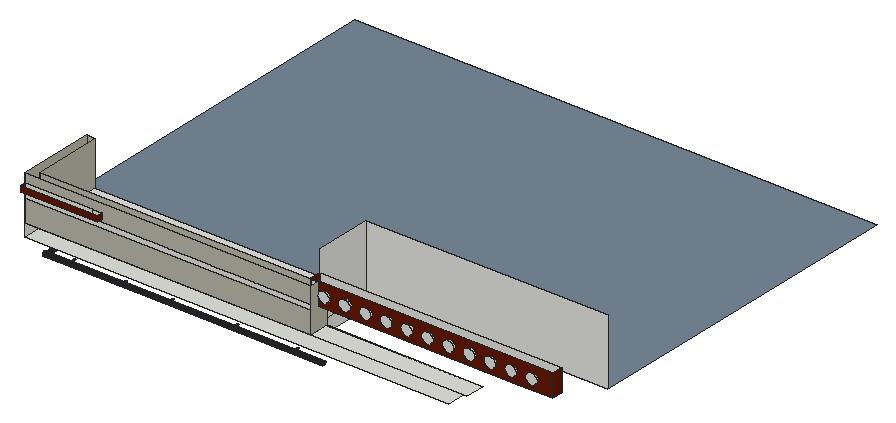
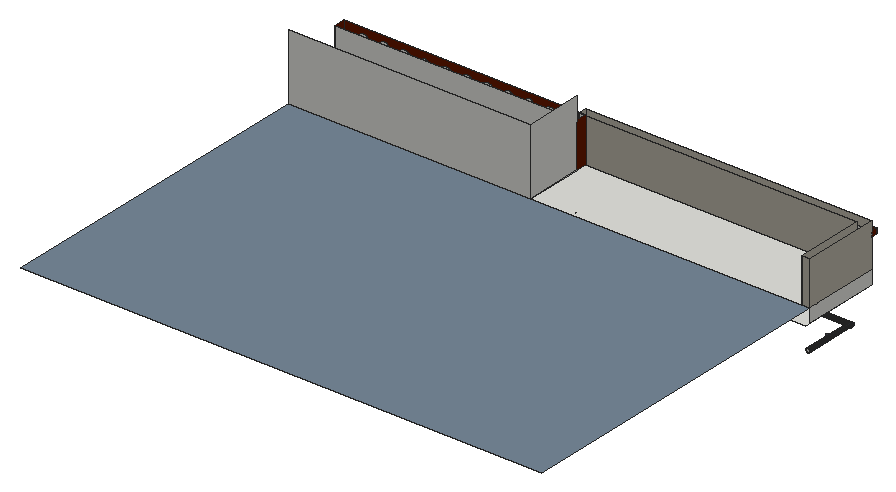
# SketchUp Ruby script. Lengths in inches.
U = 1.inch
M = Sketchup.active_model
def pt(a) = Geom::Point3d.new(a.map { |v| v * U })
def face(e, loops, mat)
  f = e.add_face(loops[0].map { |a| pt(a) })
  loops[1..].each { |l| e.add_face(l.map { |a| pt(a) }).erase! }
  f.material = f.back_material = mat if mat
  f
end
# faces: each face lists its corners as indices into pts; further lists are holes
def faces(e, pts, list, mat = nil) = list.each { |f| face(e, (f[0].is_a?(Array) ? f : [f]).map { |l| l.map { |i| pts[i] } }, mat) }
# xy, xz, yz: faces in a plane at the given z, y or x. An outline is a flat list of corners, or four numbers for a rectangle; further outlines are holes
def ring(l) = l.size == 4 ? [[l[0], l[1]], [l[2], l[1]], [l[2], l[3]], [l[0], l[3]]] : l.each_slice(2).to_a
def flat(e, list, mat, &to3) = list.each { |f| face(e, (f[0].is_a?(Array) ? f : [f]).map { |l| ring(l).map { |u, v| to3.(u, v) } }, mat) }
def xy(e, z, list, mat = nil) = flat(e, list, mat) { |x, y| [x, y, z] }
def xz(e, y, list, mat = nil) = flat(e, list, mat) { |x, z| [x, y, z] }
def yz(e, x, list, mat = nil) = flat(e, list, mat) { |y, z| [x, y, z] }
def lines(e, pts, list) = list.each { |a, b| e.add_line(pt(pts[a]), pt(pts[b])) }
# prism: a flat outline (further loops are holes) pulled along v
def prism(e, loops, v, mat = nil)
  f = face(e, loops, mat); d = Geom::Vector3d.new(v.map { |x| x * U })
  f.pushpull(f.normal.samedirection?(d) ? d.length : -d.length)
end
def box(e, o, s, mat = nil) = prism(e, [[o, [o[0] + s[0], o[1], o[2]], [o[0] + s[0], o[1] + s[1], o[2]], [o[0], o[1] + s[1], o[2]]]], [0, 0, s[2]], mat)
def at(x, y, z, deg = 0) = Geom::Transformation.translation(pt([x, y, z])) * Geom::Transformation.rotation(ORIGIN, Z_AXIS, deg.degrees)
def axes(o, x, y, z) = Geom::Transformation.new([*x, 0, *y, 0, *z, 0, *pt(o).to_a, 1])
def part(name) = M.definitions.add(name)
# library, detail: a bought-in or finely detailed component or shape, given as its bounding box
def library(name, o, s) = part(name).tap { |d| box(d.entities, o, s) }
def detail(e, o, s) = box(e.add_group.entities, o, s)
def put(e, d, t, mat = nil) = e.add_instance(d, t).tap { |i| i.material = mat if mat }
def group(e, t, mat = nil) = e.add_group.tap { |g| g.transformation = t; g.material = mat if mat }.entities
root = M.entities
M.materials.add("[0110_LightSlateGray]").color = [119, 136, 153]
M.materials.add("[0137_Black]").color = [0, 0, 0]
M.materials.add("[Color B08]").color = [102, 25, 0]
M.materials.add("[Formica Graystone]1").color = [186, 182, 168]
M.materials.add("[Formica Laminate Dark]").color = [50, 53, 60]
M.materials.add("[Wood Veneer 01]").color = [120, 70, 37]
xy(root,441.65,[[6.47,233.53,6.73,233.57,6.97,233.67,7.17,233.83,7.33,234.03,7.43,234.28,7.47,234.53,7.43,234.79,7.33,235.03,7.17,235.24,6.97,235.4,6.73,235.5,6.47,235.53,6.21,235.5,5.97,235.4,5.76,235.24,5.6,235.03,5.5,234.79,5.47,234.53,5.5,234.28,5.6,234.03,5.76,233.83,5.97,233.67,6.21,233.57]],"[Formica Laminate Dark]")
xy(root,442.09,[[91.52,203.04,91.78,203.07,92.02,203.17,92.22,203.33,92.38,203.54,92.48,203.78,92.52,204.04,92.48,204.3,92.38,204.54,92.22,204.75,92.02,204.91,91.78,205.01,91.52,205.04,91.26,205.01,91.02,204.91,90.81,204.75,90.65,204.54,90.55,204.3,90.52,204.04,90.55,203.78,90.65,203.54,90.81,203.33,91.02,203.17,91.26,203.07],[142.52,203.04,142.78,203.07,143.02,203.17,143.22,203.33,143.38,203.54,143.48,203.78,143.52,204.04,143.48,204.3,143.38,204.54,143.22,204.75,143.02,204.91,142.78,205.01,142.52,205.04,142.26,205.01,142.02,204.91,141.81,204.75,141.65,204.54,141.55,204.3,141.52,204.04,141.55,203.78,141.65,203.54,141.81,203.33,142.02,203.17,142.26,203.07],[212.89,203.04,213.15,203.07,213.39,203.17,213.6,203.33,213.76,203.54,213.86,203.78,213.89,204.04,213.86,204.3,213.76,204.54,213.6,204.75,213.39,204.91,213.15,205.01,212.89,205.04,212.63,205.01,212.39,204.91,212.18,204.75,212.03,204.54,211.93,204.3,211.89,204.04,211.93,203.78,212.03,203.54,212.18,203.33,212.39,203.17,212.63,203.07],[278.52,203.04,278.78,203.07,279.02,203.17,279.22,203.33,279.38,203.54,279.48,203.78,279.52,204.04,279.48,204.3,279.38,204.54,279.22,204.75,279.02,204.91,278.78,205.01,278.52,205.04,278.26,205.01,278.02,204.91,277.81,204.75,277.65,204.54,277.55,204.3,277.52,204.04,277.55,203.78,277.65,203.54,277.81,203.33,278.02,203.17,278.26,203.07],[34.52,204.5,34.78,204.53,35.02,204.63,35.23,204.79,35.39,205,35.49,205.24,35.52,205.5,35.49,205.76,35.39,206,35.23,206.21,35.02,206.37,34.78,206.47,34.52,206.5,34.26,206.47,34.02,206.37,33.82,206.21,33.66,206,33.56,205.76,33.52,205.5,33.56,205.24,33.66,205,33.82,204.79,34.02,204.63,34.26,204.53]],"[Formica Laminate Dark]")
xy(root,443.01,[[181.09,258.0625,209.84,261.0625],[212.72,258.0625,232.97,261.0625]])
xy(root,446.01,[[178.09,258.0625,235.97,261.0625]],"[0137_Black]")
xy(root,454.9,[[101.3,255.0625,149.3,261.0625]],"[Wood Veneer 01]")
xy(root,460.9,[[95.3,255.0625,155.3,261.0625]],"[Wood Veneer 01]")
xy(root,465.86,[[3.53,177.0625,3.53,267.0625,307.22,267.0625,307.22,198.0625,464.34,198.0625,464.34,177.0625]])
xy(root,480,[[3.53,177.0625,3.53,261.0625,12.53,261.0625,12.53,186.0625,314.59,186.0625,314.59,177.0625],[314.59,177.0625,483.9,198.0625],[12.53,186.0625,307.22,261.0625]])
xy(root,480,[[3.53,261.0625,569.78,625.1875]],"[0110_LightSlateGray]")
xy(root,504.07,[[534.65,186.0625,569.78,198.0625]])
xy(root,504.07,[[314.59,186.0625,534.65,198.0625]],"[Color B08]")
xy(root,512.39,[[3.53,171.0625,87.4,177.0625]],"[Color B08]")
xz(root,171.0625,[[3.53,512.39,87.4,518.76]],"[Color B08]")
xz(root,177.0625,[[3.53,504,314.59,509.53],[3.53,512.39,76.9,518.76],[76.9,512.39,87.4,518.76]])
xz(root,177.0625,[[3.53,480,314.59,504],[3.53,509.53,314.59,509.53,314.59,528,3.53,528,3.53,518.76,87.4,518.76,87.4,512.39,3.53,512.39]],"[Formica Graystone]1")
xz(root,183.0625,[[323.11,510.74,324.6,510.93,325.99,511.51,327.18,512.42,328.09,513.61,328.66,515,328.86,516.49,328.66,517.97,328.09,519.36,327.18,520.55,325.99,521.46,324.6,522.04,323.11,522.24,321.62,522.04,320.24,521.46,319.04,520.55,318.13,519.36,317.56,517.97,317.36,516.49,317.56,515,318.13,513.61,319.04,512.42,320.24,511.51,321.62,510.93],[345.67,510.74,347.16,510.93,348.55,511.51,349.74,512.42,350.65,513.61,351.23,515,351.42,516.49,351.23,517.97,350.65,519.36,349.74,520.55,348.55,521.46,347.16,522.04,345.67,522.24,344.19,522.04,342.8,521.46,341.61,520.55,340.69,519.36,340.12,517.97,339.92,516.49,340.12,515,340.69,513.61,341.61,512.42,342.8,511.51,344.19,510.93],[368.24,510.74,369.72,510.93,371.11,511.51,372.3,512.42,373.22,513.61,373.79,515,373.99,516.49,373.79,517.97,373.22,519.36,372.3,520.55,371.11,521.46,369.72,522.04,368.24,522.24,366.75,522.04,365.36,521.46,364.17,520.55,363.26,519.36,362.68,517.97,362.49,516.49,362.68,515,363.26,513.61,364.17,512.42,365.36,511.51,366.75,510.93],[390.8,510.74,392.29,510.93,393.67,511.51,394.86,512.42,395.78,513.61,396.35,515,396.55,516.49,396.35,517.97,395.78,519.36,394.86,520.55,393.67,521.46,392.29,522.04,390.8,522.24,389.31,522.04,387.92,521.46,386.73,520.55,385.82,519.36,385.24,517.97,385.05,516.49,385.24,515,385.82,513.61,386.73,512.42,387.92,511.51,389.31,510.93],[413.36,510.74,414.85,510.93,416.24,511.51,417.43,512.42,418.34,513.61,418.91,515,419.11,516.49,418.91,517.97,418.34,519.36,417.43,520.55,416.24,521.46,414.85,522.04,413.36,522.24,411.87,522.04,410.49,521.46,409.29,520.55,408.38,519.36,407.81,517.97,407.61,516.49,407.81,515,408.38,513.61,409.29,512.42,410.49,511.51,411.87,510.93],
  [435.92,510.74,437.41,510.93,438.8,511.51,439.99,512.42,440.9,513.61,441.48,515,441.67,516.49,441.48,517.97,440.9,519.36,439.99,520.55,438.8,521.46,437.41,522.04,435.92,522.24,434.44,522.04,433.05,521.46,431.86,520.55,430.94,519.36,430.37,517.97,430.17,516.49,430.37,515,430.94,513.61,431.86,512.42,433.05,511.51,434.44,510.93],[458.49,510.74,459.97,510.93,461.36,511.51,462.55,512.42,463.47,513.61,464.04,515,464.24,516.49,464.04,517.97,463.47,519.36,462.55,520.55,461.36,521.46,459.97,522.04,458.49,522.24,457,522.04,455.61,521.46,454.42,520.55,453.51,519.36,452.93,517.97,452.74,516.49,452.93,515,453.51,513.61,454.42,512.42,455.61,511.51,457,510.93],[481.05,510.74,482.54,510.93,483.92,511.51,485.11,512.42,486.03,513.61,486.6,515,486.8,516.49,486.6,517.97,486.03,519.36,485.11,520.55,483.92,521.46,482.54,522.04,481.05,522.24,479.56,522.04,478.17,521.46,476.98,520.55,476.07,519.36,475.49,517.97,475.3,516.49,475.49,515,476.07,513.61,476.98,512.42,478.17,511.51,479.56,510.93],[503.61,510.74,505.1,510.93,506.49,511.51,507.68,512.42,508.59,513.61,509.16,515,509.36,516.49,509.16,517.97,508.59,519.36,507.68,520.55,506.49,521.46,505.1,522.04,503.61,522.24,502.12,522.04,500.74,521.46,499.54,520.55,498.63,519.36,498.06,517.97,497.86,516.49,498.06,515,498.63,513.61,499.54,512.42,500.74,511.51,502.12,510.93],[526.17,510.74,527.66,510.93,529.05,511.51,530.24,512.42,531.15,513.61,531.73,515,531.92,516.49,531.73,517.97,531.15,519.36,530.24,520.55,529.05,521.46,527.66,522.04,526.17,522.24,524.69,522.04,523.3,521.46,522.11,520.55,521.19,519.36,520.62,517.97,520.42,516.49,520.62,515,521.19,513.61,522.11,512.42,523.3,511.51,524.69,510.93],
  [548.74,510.74,550.22,510.93,551.61,511.51,552.8,512.42,553.72,513.61,554.29,515,554.49,516.49,554.29,517.97,553.72,519.36,552.8,520.55,551.61,521.46,550.22,522.04,548.74,522.24,547.25,522.04,545.86,521.46,544.67,520.55,543.76,519.36,543.18,517.97,542.99,516.49,543.18,515,543.76,513.61,544.67,512.42,545.86,511.51,547.25,510.93]])
xz(root,186.0625,[[307.22,504.07,314.59,528],[323.11,510.74,321.62,510.93,320.24,511.51,319.04,512.42,318.13,513.61,317.56,515,317.36,516.49,317.56,517.97,318.13,519.36,319.04,520.55,320.24,521.46,321.62,522.04,323.11,522.24,324.6,522.04,325.99,521.46,327.18,520.55,328.09,519.36,328.66,517.97,328.86,516.49,328.66,515,328.09,513.61,327.18,512.42,325.99,511.51,324.6,510.93],[345.67,510.74,344.19,510.93,342.8,511.51,341.61,512.42,340.69,513.61,340.12,515,339.92,516.49,340.12,517.97,340.69,519.36,341.61,520.55,342.8,521.46,344.19,522.04,345.67,522.24,347.16,522.04,348.55,521.46,349.74,520.55,350.65,519.36,351.23,517.97,351.42,516.49,351.23,515,350.65,513.61,349.74,512.42,348.55,511.51,347.16,510.93],[368.24,510.74,366.75,510.93,365.36,511.51,364.17,512.42,363.26,513.61,362.68,515,362.49,516.49,362.68,517.97,363.26,519.36,364.17,520.55,365.36,521.46,366.75,522.04,368.24,522.24,369.72,522.04,371.11,521.46,372.3,520.55,373.22,519.36,373.79,517.97,373.99,516.49,373.79,515,373.22,513.61,372.3,512.42,371.11,511.51,369.72,510.93],[390.8,510.74,389.31,510.93,387.92,511.51,386.73,512.42,385.82,513.61,385.24,515,385.05,516.49,385.24,517.97,385.82,519.36,386.73,520.55,387.92,521.46,389.31,522.04,390.8,522.24,392.29,522.04,393.67,521.46,394.86,520.55,395.78,519.36,396.35,517.97,396.55,516.49,396.35,515,395.78,513.61,394.86,512.42,393.67,511.51,392.29,510.93],
  [413.36,510.74,411.87,510.93,410.49,511.51,409.29,512.42,408.38,513.61,407.81,515,407.61,516.49,407.81,517.97,408.38,519.36,409.29,520.55,410.49,521.46,411.87,522.04,413.36,522.24,414.85,522.04,416.24,521.46,417.43,520.55,418.34,519.36,418.91,517.97,419.11,516.49,418.91,515,418.34,513.61,417.43,512.42,416.24,511.51,414.85,510.93],[435.92,510.74,434.44,510.93,433.05,511.51,431.86,512.42,430.94,513.61,430.37,515,430.17,516.49,430.37,517.97,430.94,519.36,431.86,520.55,433.05,521.46,434.44,522.04,435.92,522.24,437.41,522.04,438.8,521.46,439.99,520.55,440.9,519.36,441.48,517.97,441.67,516.49,441.48,515,440.9,513.61,439.99,512.42,438.8,511.51,437.41,510.93],[458.49,510.74,457,510.93,455.61,511.51,454.42,512.42,453.51,513.61,452.93,515,452.74,516.49,452.93,517.97,453.51,519.36,454.42,520.55,455.61,521.46,457,522.04,458.49,522.24,459.97,522.04,461.36,521.46,462.55,520.55,463.47,519.36,464.04,517.97,464.24,516.49,464.04,515,463.47,513.61,462.55,512.42,461.36,511.51,459.97,510.93],[481.05,510.74,479.56,510.93,478.17,511.51,476.98,512.42,476.07,513.61,475.49,515,475.3,516.49,475.49,517.97,476.07,519.36,476.98,520.55,478.17,521.46,479.56,522.04,481.05,522.24,482.54,522.04,483.92,521.46,485.11,520.55,486.03,519.36,486.6,517.97,486.8,516.49,486.6,515,486.03,513.61,485.11,512.42,483.92,511.51,482.54,510.93],[503.61,510.74,502.12,510.93,500.74,511.51,499.54,512.42,498.63,513.61,498.06,515,497.86,516.49,498.06,517.97,498.63,519.36,499.54,520.55,500.74,521.46,502.12,522.04,503.61,522.24,505.1,522.04,506.49,521.46,507.68,520.55,508.59,519.36,509.16,517.97,509.36,516.49,509.16,515,508.59,513.61,507.68,512.42,506.49,511.51,505.1,510.93],
  [526.17,510.74,524.69,510.93,523.3,511.51,522.11,512.42,521.19,513.61,520.62,515,520.42,516.49,520.62,517.97,521.19,519.36,522.11,520.55,523.3,521.46,524.69,522.04,526.17,522.24,527.66,522.04,529.05,521.46,530.24,520.55,531.15,519.36,531.73,517.97,531.92,516.49,531.73,515,531.15,513.61,530.24,512.42,529.05,511.51,527.66,510.93],[548.74,510.74,547.25,510.93,545.86,511.51,544.67,512.42,543.76,513.61,543.18,515,542.99,516.49,543.18,517.97,543.76,519.36,544.67,520.55,545.86,521.46,547.25,522.04,548.74,522.24,550.22,522.04,551.61,521.46,552.8,520.55,553.72,519.36,554.29,517.97,554.49,516.49,554.29,515,553.72,513.61,552.8,512.42,551.61,511.51,550.22,510.93]])
xz(root,186.0625,[[[314.59,504.07,569.78,504.07,569.78,528.49,307.22,528.49,307.22,528,314.59,528],[548.74,510.74,547.25,510.93,545.86,511.51,544.67,512.42,543.76,513.61,543.18,515,542.99,516.49,543.18,517.97,543.76,519.36,544.67,520.55,545.86,521.46,547.25,522.04,548.74,522.24,550.22,522.04,551.61,521.46,552.8,520.55,553.72,519.36,554.29,517.97,554.49,516.49,554.29,515,553.72,513.61,552.8,512.42,551.61,511.51,550.22,510.93],[526.17,510.74,524.69,510.93,523.3,511.51,522.11,512.42,521.19,513.61,520.62,515,520.42,516.49,520.62,517.97,521.19,519.36,522.11,520.55,523.3,521.46,524.69,522.04,526.17,522.24,527.66,522.04,529.05,521.46,530.24,520.55,531.15,519.36,531.73,517.97,531.92,516.49,531.73,515,531.15,513.61,530.24,512.42,529.05,511.51,527.66,510.93],[503.61,510.74,502.12,510.93,500.74,511.51,499.54,512.42,498.63,513.61,498.06,515,497.86,516.49,498.06,517.97,498.63,519.36,499.54,520.55,500.74,521.46,502.12,522.04,503.61,522.24,505.1,522.04,506.49,521.46,507.68,520.55,508.59,519.36,509.16,517.97,509.36,516.49,509.16,515,508.59,513.61,507.68,512.42,506.49,511.51,505.1,510.93],[481.05,510.74,479.56,510.93,478.17,511.51,476.98,512.42,476.07,513.61,475.49,515,475.3,516.49,475.49,517.97,476.07,519.36,476.98,520.55,478.17,521.46,479.56,522.04,481.05,522.24,482.54,522.04,483.92,521.46,485.11,520.55,486.03,519.36,486.6,517.97,486.8,516.49,486.6,515,486.03,513.61,485.11,512.42,483.92,511.51,482.54,510.93],[458.49,510.74,457,510.93,455.61,511.51,454.42,512.42,453.51,513.61,452.93,515,452.74,516.49,452.93,517.97,453.51,519.36,454.42,520.55,455.61,521.46,457,522.04,458.49,522.24,459.97,522.04,461.36,521.46,462.55,520.55,463.47,519.36,464.04,517.97,464.24,516.49,464.04,515,463.47,513.61,462.55,512.42,461.36,511.51,459.97,510.93],[435.92,510.74,434.44,510.93,433.05,511.51,431.86,512.42,430.94,513.61,430.37,515,430.17,516.49,430.37,517.97,430.94,519.36,431.86,520.55,433.05,521.46,434.44,522.04,435.92,522.24,437.41,522.04,438.8,521.46,439.99,520.55,440.9,519.36,441.48,517.97,441.67,516.49,441.48,515,440.9,513.61,439.99,512.42,438.8,511.51,437.41,510.93],[413.36,510.74,411.87,510.93,410.49,511.51,409.29,512.42,408.38,513.61,407.81,515,407.61,516.49,407.81,517.97,408.38,519.36,409.29,520.55,410.49,521.46,411.87,522.04,413.36,522.24,414.85,522.04,416.24,521.46,417.43,520.55,418.34,519.36,418.91,517.97,419.11,516.49,418.91,515,418.34,513.61,417.43,512.42,416.24,511.51,414.85,510.93],[390.8,510.74,389.31,510.93,387.92,511.51,386.73,512.42,385.82,513.61,385.24,515,385.05,516.49,385.24,517.97,385.82,519.36,386.73,520.55,387.92,521.46,389.31,522.04,390.8,522.24,392.29,522.04,393.67,521.46,394.86,520.55,395.78,519.36,396.35,517.97,396.55,516.49,396.35,515,395.78,513.61,394.86,512.42,393.67,511.51,392.29,510.93],[368.24,510.74,366.75,510.93,365.36,511.51,364.17,512.42,363.26,513.61,362.68,515,362.49,516.49,362.68,517.97,363.26,519.36,364.17,520.55,365.36,521.46,366.75,522.04,368.24,522.24,369.72,522.04,371.11,521.46,372.3,520.55,373.22,519.36,373.79,517.97,373.99,516.49,373.79,515,373.22,513.61,372.3,512.42,371.11,511.51,369.72,510.93],[345.67,510.74,344.19,510.93,342.8,511.51,341.61,512.42,340.69,513.61,340.12,515,339.92,516.49,340.12,517.97,340.69,519.36,341.61,520.55,342.8,521.46,344.19,522.04,345.67,522.24,347.16,522.04,348.55,521.46,349.74,520.55,350.65,519.36,351.23,517.97,351.42,516.49,351.23,515,350.65,513.61,349.74,512.42,348.55,511.51,347.16,510.93],[323.11,510.74,321.62,510.93,320.24,511.51,319.04,512.42,318.13,513.61,317.56,515,317.36,516.49,317.56,517.97,318.13,519.36,319.04,520.55,320.24,521.46,321.62,522.04,323.11,522.24,324.6,522.04,325.99,521.46,327.18,520.55,328.09,519.36,328.66,517.97,328.86,516.49,328.66,515,328.09,513.61,327.18,512.42,325.99,511.51,324.6,510.93]]],"[Color B08]")
xz(root,186.0625,[[12.53,480,307.22,528]],"[Formica Graystone]1")
xz(root,198.0625,[[307.22,465.86,464.34,465.86,464.34,480,314.59,480,314.59,504.07,307.22,504.07],[307.22,504.07,569.78,528.49]])
xz(root,261.0625,[[5.64,436.11,6.21,436.18,6.74,436.4,7.1875,436.75,7.54,437.2,7.75,437.73,7.83,438.3,7.75,438.86,7.54,439.39,7.1875,439.84,6.74,440.19,6.21,440.41,5.64,440.48,5.08,440.41,4.55,440.19,4.1,439.84,3.75,439.39,3.53,438.86,3.53,437.73,3.75,437.2,4.1,436.75,4.55,436.4,5.08,436.18],[307.22,480,569.78,551.875]])
xz(root,261.0625,[[3.53,480,12.53,528]],"[Formica Graystone]1")
yz(root,3.53,[[177.0625,465.86,261.0625,480]])
yz(root,3.53,[[171.0625,512.39,177.0625,518.76]],"[Color B08]")
yz(root,3.53,[[177.0625,480,261.0625,528]],"[Formica Graystone]1")
yz(root,3.53,[[203.51,436.28,202.94,436.36,202.42,436.58,201.96,436.92,201.62,437.375,201.4,437.9,201.32,438.47,201.4,439.04,201.62,439.5625,201.96,440.02,202.42,440.36,202.94,440.58,203.51,440.66,204.08,440.58,204.6,440.36,205.06,440.02,205.41,439.5625,205.625,439.04,205.65,438.86,205.7,438.47,205.625,437.9,205.55,437.73,205.41,437.375,205.06,436.92,204.6,436.58,204.08,436.36]],"[Formica Laminate Dark]")
yz(root,12.53,[[186.0625,480,261.0625,528]],"[Formica Graystone]1")
yz(root,87.4,[[171.0625,512.39,177.0625,518.76]],"[Color B08]")
yz(root,307.22,[[198.0625,465.86,261.0625,480],[198.0625,480,261.0625,551.875]])
yz(root,307.22,[[186.0625,480,198.0625,528.49]],"[Color B08]")
yz(root,314.59,[[177.0625,480,198.0625,480,198.0625,504.07,186.0625,504.07,186.0625,528,177.0625,528]],"[Formica Graystone]1")
yz(root,569.78,[[186.0625,504.07,198.0625,528.49]],"[Color B08]")
p = [[5.08,261.0625,436.18],[5.64,261.0625,436.11],[5.64,204.08,436.11],[5.64,202.94,436.11],[5.64,202.42,436.11],[5.08,202.42,436.18],
  [6.21,261.0625,436.18],[6.21,235.5,436.18],[6.21,233.57,436.18],[6.21,202.42,436.18],[4.55,261.0625,436.4],[4.88,202.42,436.26],
  [4.73,202.42,436.33],[4.55,202.42,436.4],[6.74,261.0625,436.4],[6.74,202.42,436.4],[6.55,202.42,436.33],[6.4,202.42,436.26],
  [307.22,203.51,436.28],[307.22,202.94,436.36],[3.53,202.94,436.36],[3.53,203.51,436.28],[307.22,204.08,436.36],[3.53,204.08,436.36],
  [307.22,202.42,436.58],[6.96,202.42,436.58],[4.32,202.42,436.58],[3.53,202.42,436.58],[4.1,261.0625,436.75],[4.1,202.42,436.75],
  [7.1875,261.0625,436.75],[7.1875,202.42,436.75],[307.22,204.6,436.58],[3.53,204.6,436.58],[307.22,201.96,436.92],[3.53,201.96,436.92],
  [307.22,205.06,436.92],[3.53,205.06,436.92],[3.75,261.0625,437.2],[3.75,202.42,437.2],[7.54,261.0625,437.2],[7.54,202.42,437.2],
  [307.22,201.62,437.375],[3.53,201.62,437.375],[307.22,205.41,437.375],[3.53,205.41,437.375],[3.53,261.0625,437.73],[3.53,202.42,437.73],
  [3.53,205.55,437.73],[3.53,205.63,437.73],[3.53,205.64,437.73],[7.75,261.0625,437.73],[7.75,202.42,437.73],[307.22,201.4,437.9],
  [3.53,201.4,437.9],[307.22,205.625,437.9],[3.53,205.625,437.9],[3.45,261.0625,438.3],[3.47,202.42,438.15],[3.45,202.42,438.3],
  [7.83,261.0625,438.3],[7.83,202.42,438.3],[7.81,202.42,438.15],[307.22,201.32,438.47],[3.53,201.32,438.47],[307.22,205.7,438.47],
  [3.53,205.7,438.47],[3.53,261.0625,438.86],[3.53,202.42,438.86],[3.53,205.57,438.86],[3.53,205.59,438.86],[3.53,205.65,438.86],
  [7.75,261.0625,438.86],[7.75,202.42,438.86],[307.22,201.4,439.04],[3.53,201.4,439.04],[307.22,205.625,439.04],[3.53,205.625,439.04],
  [3.75,261.0625,439.39],[3.75,202.42,439.39],[7.54,261.0625,439.39],[7.54,202.42,439.39],[307.22,201.62,439.5625],[3.53,201.62,439.5625],
  [307.22,205.41,439.5625],[3.53,205.41,439.5625],[4.1,261.0625,439.84],[4.1,202.42,439.84],[7.1875,261.0625,439.84],[7.1875,202.42,439.84],
  [307.22,201.96,440.02],[3.53,201.96,440.02],[307.22,205.06,440.02],[3.53,205.06,440.02],[4.55,261.0625,440.19],[4.37,202.42,440.05],
  [4.45,202.42,440.11],[4.55,202.42,440.19],[6.74,261.0625,440.19],[6.74,202.42,440.19],[6.83,202.42,440.11],[6.92,202.42,440.05],
  [307.22,202.42,440.36],[6.3125,202.42,440.36],[4.97,202.42,440.36],[3.53,202.42,440.36],[307.22,204.6,440.36],[3.53,204.6,440.36],
  [5.08,261.0625,440.41],[5.08,202.42,440.41],[5.08,203.51,440.41],[6.21,261.0625,440.41],[6.21,235.5,440.41],[6.21,233.57,440.41],
  [6.21,203.51,440.41],[6.21,202.42,440.41],[307.22,202.94,440.58],[3.53,202.94,440.58],[5.64,261.0625,440.48],[5.64,202.42,440.48],
  [307.22,204.08,440.58],[3.53,204.08,440.58],[307.22,203.51,440.66],[3.53,203.51,440.66],[321.62,186.0625,510.93],[323.11,186.0625,510.74],
  [323.11,183.0625,510.74],[321.62,183.0625,510.93],[324.6,186.0625,510.93],[324.6,183.0625,510.93],[344.19,186.0625,510.93],[345.67,186.0625,510.74],
  [345.67,183.0625,510.74],[344.19,183.0625,510.93],[347.16,186.0625,510.93],[347.16,183.0625,510.93],[366.75,186.0625,510.93],[368.24,186.0625,510.74],
  [368.24,183.0625,510.74],[366.75,183.0625,510.93],[369.72,186.0625,510.93],[369.72,183.0625,510.93],[389.31,186.0625,510.93],[390.8,186.0625,510.74],
  [390.8,183.0625,510.74],[389.31,183.0625,510.93],[392.29,186.0625,510.93],[392.29,183.0625,510.93],[411.87,186.0625,510.93],[413.36,186.0625,510.74],
  [413.36,183.0625,510.74],[411.87,183.0625,510.93],[414.85,186.0625,510.93],[414.85,183.0625,510.93],[434.44,186.0625,510.93],[435.92,186.0625,510.74],
  [435.92,183.0625,510.74],[434.44,183.0625,510.93],[437.41,186.0625,510.93],[437.41,183.0625,510.93],[457,186.0625,510.93],[458.49,186.0625,510.74],
  [458.49,183.0625,510.74],[457,183.0625,510.93],[459.97,186.0625,510.93],[459.97,183.0625,510.93],[479.56,186.0625,510.93],[481.05,186.0625,510.74],
  [481.05,183.0625,510.74],[479.56,183.0625,510.93],[482.54,186.0625,510.93],[482.54,183.0625,510.93],[502.12,186.0625,510.93],[503.61,186.0625,510.74],
  [503.61,183.0625,510.74],[502.12,183.0625,510.93],[505.1,186.0625,510.93],[505.1,183.0625,510.93],[524.69,186.0625,510.93],[526.17,186.0625,510.74],
  [526.17,183.0625,510.74],[524.69,183.0625,510.93],[527.66,186.0625,510.93],[527.66,183.0625,510.93],[547.25,186.0625,510.93],[548.74,186.0625,510.74],
  [548.74,183.0625,510.74],[547.25,183.0625,510.93],[550.22,186.0625,510.93],[550.22,183.0625,510.93],[320.24,186.0625,511.51],[320.24,183.0625,511.51],
  [325.99,186.0625,511.51],[325.99,183.0625,511.51],[342.8,186.0625,511.51],[342.8,183.0625,511.51],[348.55,186.0625,511.51],[348.55,183.0625,511.51],
  [365.36,186.0625,511.51],[365.36,183.0625,511.51],[371.11,186.0625,511.51],[371.11,183.0625,511.51],[387.92,186.0625,511.51],[387.92,183.0625,511.51],
  [393.67,186.0625,511.51],[393.67,183.0625,511.51],[410.49,186.0625,511.51],[410.49,183.0625,511.51],[416.24,186.0625,511.51],[416.24,183.0625,511.51],
  [433.05,186.0625,511.51],[433.05,183.0625,511.51],[438.8,186.0625,511.51],[438.8,183.0625,511.51],[455.61,186.0625,511.51],[455.61,183.0625,511.51],
  [461.36,186.0625,511.51],[461.36,183.0625,511.51],[478.17,186.0625,511.51],[478.17,183.0625,511.51],[483.92,186.0625,511.51],[483.92,183.0625,511.51],
  [500.74,186.0625,511.51],[500.74,183.0625,511.51],[506.49,186.0625,511.51],[506.49,183.0625,511.51],[523.3,186.0625,511.51],[523.3,183.0625,511.51],
  [529.05,186.0625,511.51],[529.05,183.0625,511.51],[545.86,186.0625,511.51],[545.86,183.0625,511.51],[551.61,186.0625,511.51],[551.61,183.0625,511.51],
  [319.04,186.0625,512.42],[319.04,183.0625,512.42],[327.18,186.0625,512.42],[327.18,183.0625,512.42],[341.61,186.0625,512.42],[341.61,183.0625,512.42],
  [349.74,186.0625,512.42],[349.74,183.0625,512.42],[364.17,186.0625,512.42],[364.17,183.0625,512.42],[372.3,186.0625,512.42],[372.3,183.0625,512.42],
  [386.73,186.0625,512.42],[386.73,183.0625,512.42],[394.86,186.0625,512.42],[394.86,183.0625,512.42],[409.29,186.0625,512.42],[409.29,183.0625,512.42],
  [417.43,186.0625,512.42],[417.43,183.0625,512.42],[431.86,186.0625,512.42],[431.86,183.0625,512.42],[439.99,186.0625,512.42],[439.99,183.0625,512.42],
  [454.42,186.0625,512.42],[454.42,183.0625,512.42],[462.55,186.0625,512.42],[462.55,183.0625,512.42],[476.98,186.0625,512.42],[476.98,183.0625,512.42],
  [485.11,186.0625,512.42],[485.11,183.0625,512.42],[499.54,186.0625,512.42],[499.54,183.0625,512.42],[507.68,186.0625,512.42],[507.68,183.0625,512.42],
  [522.11,186.0625,512.42],[522.11,183.0625,512.42],[530.24,186.0625,512.42],[530.24,183.0625,512.42],[544.67,186.0625,512.42],[544.67,183.0625,512.42],
  [552.8,186.0625,512.42],[552.8,183.0625,512.42],[318.13,186.0625,513.61],[318.13,183.0625,513.61],[328.09,186.0625,513.61],[328.09,183.0625,513.61],
  [340.69,186.0625,513.61],[340.69,183.0625,513.61],[350.65,186.0625,513.61],[350.65,183.0625,513.61],[363.26,186.0625,513.61],[363.26,183.0625,513.61],
  [373.22,186.0625,513.61],[373.22,183.0625,513.61],[385.82,186.0625,513.61],[385.82,183.0625,513.61],[395.78,186.0625,513.61],[395.78,183.0625,513.61],
  [408.38,186.0625,513.61],[408.38,183.0625,513.61],[418.34,186.0625,513.61],[418.34,183.0625,513.61],[430.94,186.0625,513.61],[430.94,183.0625,513.61],
  [440.9,186.0625,513.61],[440.9,183.0625,513.61],[453.51,186.0625,513.61],[453.51,183.0625,513.61],[463.47,186.0625,513.61],[463.47,183.0625,513.61],
  [476.07,186.0625,513.61],[476.07,183.0625,513.61],[486.03,186.0625,513.61],[486.03,183.0625,513.61],[498.63,186.0625,513.61],[498.63,183.0625,513.61],
  [508.59,186.0625,513.61],[508.59,183.0625,513.61],[521.19,186.0625,513.61],[521.19,183.0625,513.61],[531.15,186.0625,513.61],[531.15,183.0625,513.61],
  [543.76,186.0625,513.61],[543.76,183.0625,513.61],[553.72,186.0625,513.61],[553.72,183.0625,513.61],[12.53,267.0625,465.86],[12.53,267.0625,480]]
faces(root,p,[[0,1,2,3,4,5],[1,6,7,8,9,4,3,2],[10,0,5,11,12,13],[6,14,15,16,17,9,8,7],[18,19,20,21],[22,18,21,23],[19,24,25,26,27,20],[28,10,13,26,29],
  [14,30,31,25,15],[32,22,23,33],[24,34,35,27,26,25],[36,32,33,37],[38,28,29,39],[30,40,41,31],[34,42,43,35],[44,36,37,45],
  [46,38,39,47,48,49,50],[40,51,52,41],[42,53,54,43],[55,44,45,48,56],[57,46,50,49,48,47,58,59],[51,60,61,62,52],[53,63,64,54],[65,55,56,66],
  [67,57,59,68,69,70,71],[60,72,73,61],[63,74,75,64],[76,65,66,71,77],[78,67,71,70,69,68,79],[72,80,81,73],[74,82,83,75],[84,76,77,85],
  [86,78,79,87],[80,88,89,81],[82,90,91,83],[92,84,85,93],[94,86,87,95,96,97],[88,98,99,100,101,89],[90,102,103,104,105,91],[106,92,93,107],
  [108,94,97,104,109,110],[98,111,112,113,114,115,103,99],[102,116,117,105,104,103],[118,108,110,109,119],[111,118,119,115,114,113,112],[120,106,107,121],[116,122,123,117],[122,120,121,123]],"[Formica Laminate Dark]")
faces(root,p,[[124,125,126,127],[125,128,129,126],[130,131,132,133],[131,134,135,132],[136,137,138,139],[137,140,141,138],[142,143,144,145],[143,146,147,144],
  [148,149,150,151],[149,152,153,150],[154,155,156,157],[155,158,159,156],[160,161,162,163],[161,164,165,162],[166,167,168,169],[167,170,171,168],
  [172,173,174,175],[173,176,177,174],[178,179,180,181],[179,182,183,180],[184,185,186,187],[185,188,189,186],[190,124,127,191],[128,192,193,129],
  [194,130,133,195],[134,196,197,135],[198,136,139,199],[140,200,201,141],[202,142,145,203],[146,204,205,147],[206,148,151,207],[152,208,209,153],
  [210,154,157,211],[158,212,213,159],[214,160,163,215],[164,216,217,165],[218,166,169,219],[170,220,221,171],[222,172,175,223],[176,224,225,177],
  [226,178,181,227],[182,228,229,183],[230,184,187,231],[188,232,233,189],[234,190,191,235],[192,236,237,193],[238,194,195,239],[196,240,241,197],
  [242,198,199,243],[200,244,245,201],[246,202,203,247],[204,248,249,205],[250,206,207,251],[208,252,253,209],[254,210,211,255],[212,256,257,213],
  [258,214,215,259],[216,260,261,217],[262,218,219,263],[220,264,265,221],[266,222,223,267],[224,268,269,225],[270,226,227,271],[228,272,273,229],
  [274,230,231,275],[232,276,277,233],[278,234,235,279],[236,280,281,237],[282,238,239,283],[240,284,285,241],[286,242,243,287],[244,288,289,245],
  [290,246,247,291],[248,292,293,249],[294,250,251,295],[252,296,297,253],[298,254,255,299],[256,300,301,257],[302,258,259,303],[260,304,305,261],
  [306,262,263,307],[264,308,309,265],[310,266,267,311],[268,312,313,269],[314,270,271,315],[272,316,317,273],[318,274,275,319],[276,320,321,277]])
lines(root,p,[[322,323]])
